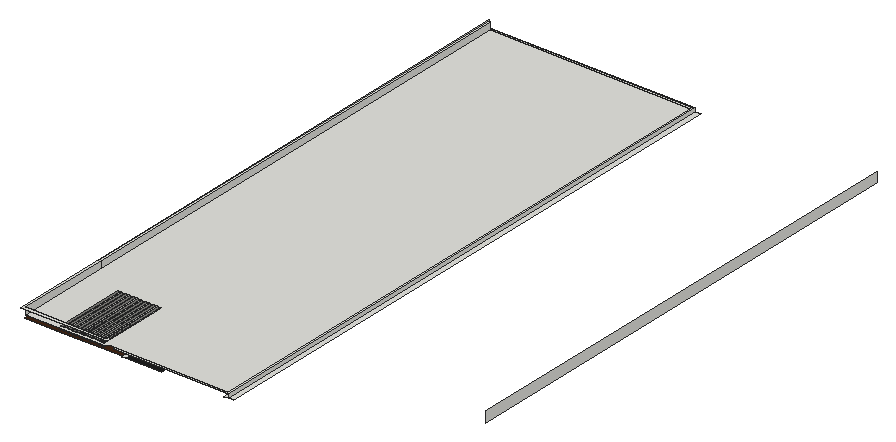
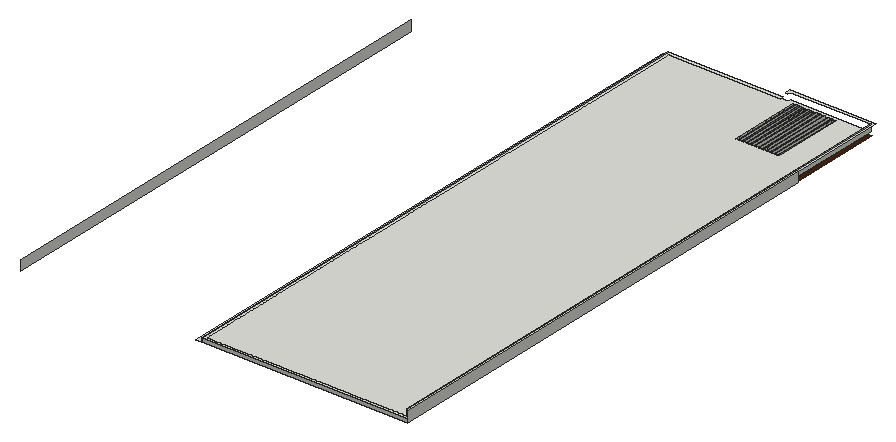
# SketchUp Ruby script. Lengths in inches.
U = 1.inch
M = Sketchup.active_model
def pt(a) = Geom::Point3d.new(a.map { |v| v * U })
def face(e, loops, mat)
  f = e.add_face(loops[0].map { |a| pt(a) })
  loops[1..].each { |l| e.add_face(l.map { |a| pt(a) }).erase! }
  f.material = f.back_material = mat if mat
  f
end
# faces: each face lists its corners as indices into pts; further lists are holes
def faces(e, pts, list, mat = nil) = list.each { |f| face(e, (f[0].is_a?(Array) ? f : [f]).map { |l| l.map { |i| pts[i] } }, mat) }
# xy, xz, yz: faces in a plane at the given z, y or x. An outline is a flat list of corners, or four numbers for a rectangle; further outlines are holes
def ring(l) = l.size == 4 ? [[l[0], l[1]], [l[2], l[1]], [l[2], l[3]], [l[0], l[3]]] : l.each_slice(2).to_a
def flat(e, list, mat, &to3) = list.each { |f| face(e, (f[0].is_a?(Array) ? f : [f]).map { |l| ring(l).map { |u, v| to3.(u, v) } }, mat) }
def xy(e, z, list, mat = nil) = flat(e, list, mat) { |x, y| [x, y, z] }
def xz(e, y, list, mat = nil) = flat(e, list, mat) { |x, z| [x, y, z] }
def yz(e, x, list, mat = nil) = flat(e, list, mat) { |y, z| [x, y, z] }
def lines(e, pts, list) = list.each { |a, b| e.add_line(pt(pts[a]), pt(pts[b])) }
# prism: a flat outline (further loops are holes) pulled along v
def prism(e, loops, v, mat = nil)
  f = face(e, loops, mat); d = Geom::Vector3d.new(v.map { |x| x * U })
  f.pushpull(f.normal.samedirection?(d) ? d.length : -d.length)
end
def box(e, o, s, mat = nil) = prism(e, [[o, [o[0] + s[0], o[1], o[2]], [o[0] + s[0], o[1] + s[1], o[2]], [o[0], o[1] + s[1], o[2]]]], [0, 0, s[2]], mat)
def at(x, y, z, deg = 0) = Geom::Transformation.translation(pt([x, y, z])) * Geom::Transformation.rotation(ORIGIN, Z_AXIS, deg.degrees)
def axes(o, x, y, z) = Geom::Transformation.new([*x, 0, *y, 0, *z, 0, *pt(o).to_a, 1])
def part(name) = M.definitions.add(name)
# library, detail: a bought-in or finely detailed component or shape, given as its bounding box
def library(name, o, s) = part(name).tap { |d| box(d.entities, o, s) }
def detail(e, o, s) = box(e.add_group.entities, o, s)
def put(e, d, t, mat = nil) = e.add_instance(d, t).tap { |i| i.material = mat if mat }
def group(e, t, mat = nil) = e.add_group.tap { |g| g.transformation = t; g.material = mat if mat }.entities
root = M.entities
M.materials.add("[Color M08]").color = [30, 30, 30]
M.materials.add("[Field Square Tile]").color = [211, 167, 108]
M.materials.add("[Granite Light Gray]").color = [149, 148, 144]
M.materials.add("[Wood Veneer 01]").color = [66, 38, 20]
xy(root,380.5,[[2434.04,2346.71,2434.04,3661.44,1986.28,3661.44,1986.28,2597.8,2202.28,2597.8,2202.28,2562.82,1976.47,2562.82,1976.47,3671.25,2443.85,3671.25,2443.85,2346.71],[2202.28,2346.71,2211.2,2425.46],[2443.85,2346.71,2455.66,3671.25],[2202.28,2425.46,2202.28,2597.8,1986.28,2597.8,1986.28,3661.44,2434.04,3661.44,2434.04,2425.46,2387.27,2425.46,2387.27,2532.83,2291.96,2532.83,2291.96,2573.65,2211.2,2573.65,2211.2,2532.83,2202.58,2532.83,2202.58,2425.46],[2202.58,2425.46,2211.2,2532.83],
  [2291.96,2425.46,2387.27,2532.83],[2211.2,2532.83,2291.96,2573.65]])
xy(root,380.5,[[2211.2,2346.71,2291.96,2532.83]],"[Color M08]")
xy(root,380.5,[[[1981.3,2347.9,2053.23,2562.82],[2038.08,2501.63,2039.6,2502.01,2040.98,2502.76,2042.11,2503.84,2042.92,2505.18,2043.35,2506.6875,2043.39,2508.25,2043.01,2509.78,2042.26,2511.15,2041.17,2512.28,2039.83,2513.09,2038.33,2513.53,2036.76,2513.56,2035.24,2513.19,2033.87,2512.43,2032.74,2511.35,2031.93,2510.01,2031.49,2508.5,2031.46,2506.9375,2031.83,2505.41,2032.59,2504.04,2033.67,2502.91,2035.01,2502.1,2036.52,2501.66],[2038.08,2441.63,2039.6,2442.01,2040.98,2442.76,2042.11,2443.84,2042.92,2445.18,2043.35,2446.6875,2043.39,2448.25,2043.01,2449.78,2042.26,2451.15,2041.17,2452.28,2039.83,2453.09,2038.33,2453.53,2036.76,2453.56,2035.24,2453.19,2033.87,2452.43,2032.74,2451.35,2031.93,2450.01,2031.49,2448.5,2031.46,2446.9375,2031.83,2445.41,2032.59,2444.04,2033.67,2442.91,2035.01,2442.1,2036.52,2441.66],[2038.08,2389.88,2039.6,2390.26,2040.98,2391.01,2042.11,2392.09,2042.92,2393.43,2043.35,2394.9375,2043.39,2396.5,2043.01,2398.03,2042.26,2399.4,2041.17,2400.53,2039.83,2401.34,2038.33,2401.78,2036.76,2401.81,2035.24,2401.44,2033.87,2400.68,2032.74,2399.6,2031.93,2398.26,2031.49,2396.75,2031.46,2395.1875,2031.83,2393.66,2032.59,2392.29,2033.67,2391.16,2035.01,2390.35,2036.52,2389.91],[2038.08,2359.13,2039.6,2359.51,2040.98,2360.26,2042.11,2361.34,2042.92,2362.68,2043.35,2364.1875,2043.39,2365.75,2043.01,2367.28,2042.26,2368.65,2041.17,2369.78,2039.83,2370.59,2038.33,2371.03,2036.76,2371.06,2035.24,2370.69,2033.87,2369.93,2032.74,2368.85,2031.93,2367.51,2031.49,2366,2031.46,2364.4375,2031.83,2362.91,2032.59,2361.54,2033.67,2360.41,2035.01,2359.6,2036.52,2359.16],[1998.33,2501.63,1999.85,2502.01,2001.23,2502.76,2002.36,2503.84,2003.17,2505.18,2003.6,2506.6875,2003.64,2508.25,2003.26,2509.78,2002.51,2511.15,2001.42,2512.28,2000.08,2513.09,1998.58,2513.53,1997.01,2513.56,1995.49,2513.19,1994.12,2512.43,1992.99,2511.35,1992.18,2510.01,1991.74,2508.5,1991.71,2506.9375,1992.08,2505.41,1992.84,2504.04,1993.92,2502.91,1995.26,2502.1,1996.77,2501.66],[1998.33,2441.63,1999.85,2442.01,2001.23,2442.76,2002.36,2443.84,2003.17,2445.18,2003.6,2446.6875,2003.64,2448.25,2003.26,2449.78,2002.51,2451.15,2001.42,2452.28,2000.08,2453.09,1998.58,2453.53,1997.01,2453.56,1995.49,2453.19,1994.12,2452.43,1992.99,2451.35,1992.18,2450.01,1991.74,2448.5,1991.71,2446.9375,1992.08,2445.41,1992.84,2444.04,1993.92,2442.91,1995.26,2442.1,1996.77,2441.66],[1998.33,2389.88,1999.85,2390.26,2001.23,2391.01,2002.36,2392.09,2003.17,2393.43,2003.6,2394.9375,2003.64,2396.5,2003.26,2398.03,2002.51,2399.4,2001.42,2400.53,2000.08,2401.34,1998.58,2401.78,1997.01,2401.81,1995.49,2401.44,1994.12,2400.68,1992.99,2399.6,1992.18,2398.26,1991.74,2396.75,1991.71,2395.1875,1992.08,2393.66,1992.84,2392.29,1993.92,2391.16,1995.26,2390.35,1996.77,2389.91],[1998.33,2359.13,1999.85,2359.51,2001.23,2360.26,2002.36,2361.34,2003.17,2362.68,2003.6,2364.1875,2003.64,2365.75,2003.26,2367.28,2002.51,2368.65,2001.42,2369.78,2000.08,2370.59,1998.58,2371.03,1997.01,2371.06,1995.49,2370.69,1994.12,2369.93,1992.99,2368.85,1992.18,2367.51,1991.74,2366,1991.71,2364.4375,1992.08,2362.91,1992.84,2361.54,1993.92,2360.41,1995.26,2359.6,1996.77,2359.16]],[[2053.23,2347.9,2202.28,2562.82],[2148.68,2355.06,2154.93,2516.12],[2139.56,2355.06,2145.81,2516.12],[2130.43,2355.06,2136.68,2516.12],[2121.31,2355.06,2127.56,2516.12],[2112.18,2355.06,2118.43,2516.12],[2103.06,2355.06,2109.31,2516.12],[2093.93,2355.06,2100.18,2516.12],[2084.81,2355.06,2091.06,2516.12],[2075.68,2355.06,2081.93,2516.12],[2066.56,2355.06,2072.81,2516.12],[2057.43,2355.06,2063.68,2516.12]]],"[Wood Veneer 01]")
xy(root,381.875,[[1998.33,2389.88,1996.77,2389.91,1995.26,2390.35,1993.92,2391.16,1992.84,2392.29,1992.08,2393.66,1991.71,2395.1875,1991.74,2396.75,1992.18,2398.26,1992.99,2399.6,1994.12,2400.68,1995.49,2401.44,1997.01,2401.81,1998.58,2401.78,2000.08,2401.34,2001.42,2400.53,2002.51,2399.4,2003.26,2398.03,2003.64,2396.5,2003.6,2394.9375,2003.17,2393.43,2002.36,2392.09,2001.23,2391.01,1999.85,2390.26],[2038.08,2389.88,2036.52,2389.91,2035.01,2390.35,2033.67,2391.16,2032.59,2392.29,2031.83,2393.66,2031.46,2395.1875,2031.49,2396.75,2031.93,2398.26,2032.74,2399.6,2033.87,2400.68,2035.24,2401.44,2036.76,2401.81,2038.33,2401.78,2039.83,2401.34,2041.17,2400.53,2042.26,2399.4,2043.01,2398.03,2043.39,2396.5,2043.35,2394.9375,2042.92,2393.43,2042.11,2392.09,2040.98,2391.01,2039.6,2390.26],[1998.33,2441.63,1996.77,2441.66,1995.26,2442.1,1993.92,2442.91,1992.84,2444.04,1992.08,2445.41,1991.71,2446.9375,1991.74,2448.5,1992.18,2450.01,1992.99,2451.35,1994.12,2452.43,1995.49,2453.19,1997.01,2453.56,1998.58,2453.53,2000.08,2453.09,2001.42,2452.28,2002.51,2451.15,2003.26,2449.78,2003.64,2448.25,2003.6,2446.6875,2003.17,2445.18,2002.36,2443.84,2001.23,2442.76,1999.85,2442.01],[2038.08,2441.63,2036.52,2441.66,2035.01,2442.1,2033.67,2442.91,2032.59,2444.04,2031.83,2445.41,2031.46,2446.9375,2031.49,2448.5,2031.93,2450.01,2032.74,2451.35,2033.87,2452.43,2035.24,2453.19,2036.76,2453.56,2038.33,2453.53,2039.83,2453.09,2041.17,2452.28,2042.26,2451.15,2043.01,2449.78,2043.39,2448.25,2043.35,2446.6875,2042.92,2445.18,2042.11,2443.84,2040.98,2442.76,2039.6,2442.01],[1998.33,2501.63,1996.77,2501.66,1995.26,2502.1,1993.92,2502.91,1992.84,2504.04,1992.08,2505.41,1991.71,2506.9375,1991.74,2508.5,1992.18,2510.01,1992.99,2511.35,1994.12,2512.43,1995.49,2513.19,1997.01,2513.56,1998.58,2513.53,2000.08,2513.09,2001.42,2512.28,2002.51,2511.15,2003.26,2509.78,2003.64,2508.25,2003.6,2506.6875,2003.17,2505.18,2002.36,2503.84,2001.23,2502.76,1999.85,2502.01],
  [2038.08,2501.63,2036.52,2501.66,2035.01,2502.1,2033.67,2502.91,2032.59,2504.04,2031.83,2505.41,2031.46,2506.9375,2031.49,2508.5,2031.93,2510.01,2032.74,2511.35,2033.87,2512.43,2035.24,2513.19,2036.76,2513.56,2038.33,2513.53,2039.83,2513.09,2041.17,2512.28,2042.26,2511.15,2043.01,2509.78,2043.39,2508.25,2043.35,2506.6875,2042.92,2505.18,2042.11,2503.84,2040.98,2502.76,2039.6,2502.01]],"[Field Square Tile]")
xy(root,388.625,[[[1982.81,2346.49,2166.13,2346.49,2166.13,2353.05,2437.5,2353.05,2437.5,3664.91,1982.81,3664.91],[2057.43,2355.06,2063.68,2516.12],[2066.56,2355.06,2072.81,2516.12],[2075.68,2355.06,2081.93,2516.12],[2084.81,2355.06,2091.06,2516.12],[2093.93,2355.06,2100.18,2516.12],[2103.06,2355.06,2109.31,2516.12],[2112.18,2355.06,2118.43,2516.12],[2121.31,2355.06,2127.56,2516.12],[2130.43,2355.06,2136.68,2516.12],[2139.56,2355.06,2145.81,2516.12],[2148.68,2355.06,2154.93,2516.12]],[2183.1875,2346.71,2443.85,2346.71,2443.85,3671.25,1976.47,3671.25,1982.81,3664.91,2437.5,3664.91,2437.5,2353.05,2183.1875,2353.05]])
xy(root,403.8125,[[1976.47,2340.15,2172.48,2340.15,2172.48,2353.05,2166.13,2353.05,2166.13,2346.49,1982.81,2346.49,1982.81,3664.91,1976.47,3671.25]])
xz(root,2516.12,[[2057.43,380.5,2063.68,388.625],[2066.56,380.5,2072.81,388.625],[2075.68,380.5,2081.93,388.625],[2084.81,380.5,2091.06,388.625],[2093.93,380.5,2100.18,388.625],
  [2103.06,380.5,2109.31,388.625],[2112.18,380.5,2118.43,388.625],[2121.31,380.5,2127.56,388.625],[2130.43,380.5,2136.68,388.625],[2139.56,380.5,2145.81,388.625],
  [2148.68,380.5,2154.93,388.625]],"[Granite Light Gray]")
xz(root,3671.25,[[1976.47,380.5,2443.85,388.625]])
yz(root,1976.47,[[2562.82,380.5,3671.25,403.8125]])
yz(root,1982.81,[[2346.49,388.625,2562.82,403.8125],[2562.82,388.625,3664.91,403.8125]])
yz(root,2057.43,[[2355.06,380.5,2516.12,388.625]],"[Granite Light Gray]")
yz(root,2063.68,[[2355.06,380.5,2516.12,388.625]])
yz(root,2066.56,[[2355.06,380.5,2516.12,388.625]],"[Granite Light Gray]")
yz(root,2072.81,[[2355.06,380.5,2516.12,388.625]])
yz(root,2075.68,[[2355.06,380.5,2516.12,388.625]],"[Granite Light Gray]")
yz(root,2081.93,[[2355.06,380.5,2516.12,388.625]])
yz(root,2084.81,[[2355.06,380.5,2516.12,388.625]],"[Granite Light Gray]")
yz(root,2091.06,[[2355.06,380.5,2516.12,388.625]])
yz(root,2093.93,[[2355.06,380.5,2516.12,388.625]],"[Granite Light Gray]")
yz(root,2100.18,[[2355.06,380.5,2516.12,388.625]])
yz(root,2103.06,[[2355.06,380.5,2516.12,388.625]],"[Granite Light Gray]")
yz(root,2109.31,[[2355.06,380.5,2516.12,388.625]])
yz(root,2112.18,[[2355.06,380.5,2516.12,388.625]],"[Granite Light Gray]")
yz(root,2118.43,[[2355.06,380.5,2516.12,388.625]])
yz(root,2121.31,[[2355.06,380.5,2516.12,388.625]],"[Granite Light Gray]")
yz(root,2127.56,[[2355.06,380.5,2516.12,388.625]])
yz(root,2130.43,[[2355.06,380.5,2516.12,388.625]],"[Granite Light Gray]")
yz(root,2136.68,[[2355.06,380.5,2516.12,388.625]])
yz(root,2139.56,[[2355.06,380.5,2516.12,388.625]],"[Granite Light Gray]")
yz(root,2145.81,[[2355.06,380.5,2516.12,388.625]])
yz(root,2148.68,[[2355.06,380.5,2516.12,388.625]],"[Granite Light Gray]")
yz(root,2154.93,[[2355.06,380.5,2516.12,388.625]])
yz(root,2443.85,[[2346.71,380.5,3671.25,388.625]])
yz(root,2855.22,[[2562.82,380.5,3671.25,403.8125]])
p = [[1996.77,2389.91,380.5],[1995.26,2390.35,380.5],[1995.26,2390.35,381.875],[1996.77,2389.91,381.875],[1998.33,2389.88,380.5],[1998.33,2389.88,381.875],
  [1999.85,2390.26,380.5],[1999.85,2390.26,381.875],[2036.52,2389.91,380.5],[2035.01,2390.35,380.5],[2035.01,2390.35,381.875],[2036.52,2389.91,381.875],
  [2038.08,2389.88,380.5],[2038.08,2389.88,381.875],[2039.6,2390.26,380.5],[2039.6,2390.26,381.875],[2001.23,2391.01,380.5],[2001.23,2391.01,381.875],
  [2040.98,2391.01,380.5],[2040.98,2391.01,381.875],[1993.92,2391.16,380.5],[1993.92,2391.16,381.875],[2033.67,2391.16,380.5],[2033.67,2391.16,381.875],
  [2002.36,2392.09,380.5],[2002.36,2392.09,381.875],[2042.11,2392.09,380.5],[2042.11,2392.09,381.875],[1992.84,2392.29,380.5],[1992.84,2392.29,381.875],
  [2032.59,2392.29,380.5],[2032.59,2392.29,381.875],[2003.17,2393.43,380.5],[2003.17,2393.43,381.875],[2042.92,2393.43,380.5],[2042.92,2393.43,381.875],
  [1992.08,2393.66,380.5],[1992.08,2393.66,381.875],[2031.83,2393.66,380.5],[2031.83,2393.66,381.875],[2003.6,2394.9375,380.5],[2003.6,2394.9375,381.875],
  [2043.35,2394.9375,380.5],[2043.35,2394.9375,381.875],[1991.71,2395.1875,380.5],[1991.71,2395.1875,381.875],[2031.46,2395.1875,380.5],[2031.46,2395.1875,381.875],
  [2003.64,2396.5,380.5],[2003.64,2396.5,381.875],[2043.39,2396.5,380.5],[2043.39,2396.5,381.875],[1991.74,2396.75,380.5],[1991.74,2396.75,381.875],
  [2031.49,2396.75,380.5],[2031.49,2396.75,381.875],[2003.26,2398.03,380.5],[2003.26,2398.03,381.875],[2043.01,2398.03,380.5],[2043.01,2398.03,381.875],
  [1992.18,2398.26,380.5],[1992.18,2398.26,381.875],[2031.93,2398.26,380.5],[2031.93,2398.26,381.875],[2002.51,2399.4,380.5],[2002.51,2399.4,381.875],
  [2042.26,2399.4,380.5],[2042.26,2399.4,381.875],[1992.99,2399.6,380.5],[1992.99,2399.6,381.875],[2032.74,2399.6,380.5],[2032.74,2399.6,381.875],
  [2001.42,2400.53,380.5],[2001.42,2400.53,381.875],[2041.17,2400.53,380.5],[2041.17,2400.53,381.875],[1994.12,2400.68,380.5],[1994.12,2400.68,381.875],
  [2033.87,2400.68,380.5],[2033.87,2400.68,381.875],[2000.08,2401.34,380.5],[2000.08,2401.34,381.875],[2039.83,2401.34,380.5],[2039.83,2401.34,381.875],
  [1995.49,2401.44,380.5],[1995.49,2401.44,381.875],[2035.24,2401.44,380.5],[2035.24,2401.44,381.875],[1998.58,2401.78,380.5],[1998.58,2401.78,381.875],
  [2038.33,2401.78,380.5],[2038.33,2401.78,381.875],[1997.01,2401.81,380.5],[1997.01,2401.81,381.875],[2036.76,2401.81,380.5],[2036.76,2401.81,381.875],
  [1998.33,2441.63,380.5],[1996.77,2441.66,380.5],[1996.77,2441.66,381.875],[1998.33,2441.63,381.875],[1999.85,2442.01,380.5],[1999.85,2442.01,381.875],
  [2038.08,2441.63,380.5],[2036.52,2441.66,380.5],[2036.52,2441.66,381.875],[2038.08,2441.63,381.875],[2039.6,2442.01,380.5],[2039.6,2442.01,381.875],
  [1995.26,2442.1,380.5],[1995.26,2442.1,381.875],[2035.01,2442.1,380.5],[2035.01,2442.1,381.875],[2001.23,2442.76,380.5],[2001.23,2442.76,381.875],
  [2040.98,2442.76,380.5],[2040.98,2442.76,381.875],[1993.92,2442.91,380.5],[1993.92,2442.91,381.875],[2033.67,2442.91,380.5],[2033.67,2442.91,381.875],
  [2002.36,2443.84,380.5],[2002.36,2443.84,381.875],[2042.11,2443.84,380.5],[2042.11,2443.84,381.875],[1992.84,2444.04,380.5],[1992.84,2444.04,381.875],
  [2032.59,2444.04,380.5],[2032.59,2444.04,381.875],[2003.17,2445.18,380.5],[2003.17,2445.18,381.875],[2042.92,2445.18,380.5],[2042.92,2445.18,381.875],
  [1992.08,2445.41,380.5],[1992.08,2445.41,381.875],[2031.83,2445.41,380.5],[2031.83,2445.41,381.875],[2003.6,2446.6875,380.5],[2003.6,2446.6875,381.875],
  [2043.35,2446.6875,380.5],[2043.35,2446.6875,381.875],[1991.71,2446.9375,380.5],[1991.71,2446.9375,381.875],[2031.46,2446.9375,380.5],[2031.46,2446.9375,381.875],
  [2003.64,2448.25,380.5],[2003.64,2448.25,381.875],[2043.39,2448.25,380.5],[2043.39,2448.25,381.875],[1991.74,2448.5,380.5],[1991.74,2448.5,381.875],
  [2031.49,2448.5,380.5],[2031.49,2448.5,381.875],[2003.26,2449.78,380.5],[2003.26,2449.78,381.875],[2043.01,2449.78,380.5],[2043.01,2449.78,381.875],
  [1992.18,2450.01,380.5],[1992.18,2450.01,381.875],[2031.93,2450.01,380.5],[2031.93,2450.01,381.875],[2002.51,2451.15,380.5],[2002.51,2451.15,381.875],
  [2042.26,2451.15,380.5],[2042.26,2451.15,381.875],[1992.99,2451.35,380.5],[1992.99,2451.35,381.875],[2032.74,2451.35,380.5],[2032.74,2451.35,381.875],
  [2001.42,2452.28,380.5],[2001.42,2452.28,381.875],[2041.17,2452.28,380.5],[2041.17,2452.28,381.875],[1994.12,2452.43,380.5],[1994.12,2452.43,381.875],
  [2033.87,2452.43,380.5],[2033.87,2452.43,381.875],[2000.08,2453.09,380.5],[2000.08,2453.09,381.875],[2039.83,2453.09,380.5],[2039.83,2453.09,381.875],
  [1995.49,2453.19,380.5],[1995.49,2453.19,381.875],[2035.24,2453.19,380.5],[2035.24,2453.19,381.875],[1998.58,2453.53,380.5],[1998.58,2453.53,381.875],
  [2038.33,2453.53,380.5],[2038.33,2453.53,381.875],[1997.01,2453.56,380.5],[1997.01,2453.56,381.875],[2036.76,2453.56,380.5],[2036.76,2453.56,381.875],
  [1998.33,2501.63,380.5],[1996.77,2501.66,380.5],[1996.77,2501.66,381.875],[1998.33,2501.63,381.875],[1999.85,2502.01,380.5],[1999.85,2502.01,381.875],
  [2038.08,2501.63,380.5],[2036.52,2501.66,380.5],[2036.52,2501.66,381.875],[2038.08,2501.63,381.875],[2039.6,2502.01,380.5],[2039.6,2502.01,381.875],
  [1995.26,2502.1,380.5],[1995.26,2502.1,381.875],[2035.01,2502.1,380.5],[2035.01,2502.1,381.875],[2001.23,2502.76,380.5],[2001.23,2502.76,381.875],
  [2040.98,2502.76,380.5],[2040.98,2502.76,381.875],[1993.92,2502.91,380.5],[1993.92,2502.91,381.875],[2033.67,2502.91,380.5],[2033.67,2502.91,381.875],
  [2002.36,2503.84,380.5],[2002.36,2503.84,381.875],[2042.11,2503.84,380.5],[2042.11,2503.84,381.875],[1992.84,2504.04,380.5],[1992.84,2504.04,381.875],
  [2032.59,2504.04,380.5],[2032.59,2504.04,381.875],[2003.17,2505.18,380.5],[2003.17,2505.18,381.875],[2042.92,2505.18,380.5],[2042.92,2505.18,381.875],
  [1992.08,2505.41,380.5],[1992.08,2505.41,381.875],[2031.83,2505.41,380.5],[2031.83,2505.41,381.875],[2003.6,2506.6875,380.5],[2003.6,2506.6875,381.875],
  [2043.35,2506.6875,380.5],[2043.35,2506.6875,381.875],[1991.71,2506.9375,380.5],[1991.71,2506.9375,381.875],[2031.46,2506.9375,380.5],[2031.46,2506.9375,381.875],
  [2003.64,2508.25,380.5],[2003.64,2508.25,381.875],[2043.39,2508.25,380.5],[2043.39,2508.25,381.875],[1991.74,2508.5,380.5],[1991.74,2508.5,381.875],
  [2031.49,2508.5,380.5],[2031.49,2508.5,381.875],[2003.26,2509.78,380.5],[2003.26,2509.78,381.875],[2043.01,2509.78,380.5],[2043.01,2509.78,381.875],
  [1992.18,2510.01,380.5],[1992.18,2510.01,381.875],[2031.93,2510.01,380.5],[2031.93,2510.01,381.875],[2002.51,2511.15,380.5],[2002.51,2511.15,381.875],
  [2042.26,2511.15,380.5],[2042.26,2511.15,381.875],[1992.99,2511.35,380.5],[1992.99,2511.35,381.875],[2032.74,2511.35,380.5],[2032.74,2511.35,381.875],
  [2001.42,2512.28,380.5],[2001.42,2512.28,381.875],[2041.17,2512.28,380.5],[2041.17,2512.28,381.875],[1994.12,2512.43,380.5],[1994.12,2512.43,381.875],
  [2033.87,2512.43,380.5],[2033.87,2512.43,381.875],[2000.08,2513.09,380.5],[2000.08,2513.09,381.875],[2039.83,2513.09,380.5],[2039.83,2513.09,381.875],
  [1995.49,2513.19,380.5],[1995.49,2513.19,381.875],[2035.24,2513.19,380.5],[2035.24,2513.19,381.875],[1998.58,2513.53,380.5],[1998.58,2513.53,381.875],
  [2038.33,2513.53,380.5],[2038.33,2513.53,381.875],[1997.01,2513.56,380.5],[1997.01,2513.56,381.875],[2036.76,2513.56,380.5],[2036.76,2513.56,381.875],
  [1982.81,3664.91,388.625],[1976.47,3671.25,388.625],[1976.47,3671.25,403.8125],[1982.81,3664.91,403.8125]]
faces(root,p,[[0,1,2,3],[4,0,3,5],[6,4,5,7],[8,9,10,11],[12,8,11,13],[14,12,13,15],[16,6,7,17],[18,14,15,19],
  [1,20,21,2],[9,22,23,10],[24,16,17,25],[26,18,19,27],[20,28,29,21],[22,30,31,23],[32,24,25,33],[34,26,27,35],
  [28,36,37,29],[30,38,39,31],[40,32,33,41],[42,34,35,43],[36,44,45,37],[38,46,47,39],[48,40,41,49],[50,42,43,51],
  [44,52,53,45],[46,54,55,47],[56,48,49,57],[58,50,51,59],[52,60,61,53],[54,62,63,55],[64,56,57,65],[66,58,59,67],
  [60,68,69,61],[62,70,71,63],[72,64,65,73],[74,66,67,75],[68,76,77,69],[70,78,79,71],[80,72,73,81],[82,74,75,83],
  [76,84,85,77],[78,86,87,79],[88,80,81,89],[90,82,83,91],[84,92,93,85],[86,94,95,87],[92,88,89,93],[94,90,91,95],
  [96,97,98,99],[100,96,99,101],[102,103,104,105],[106,102,105,107],[97,108,109,98],[103,110,111,104],[112,100,101,113],[114,106,107,115],
  [108,116,117,109],[110,118,119,111],[120,112,113,121],[122,114,115,123],[116,124,125,117],[118,126,127,119],[128,120,121,129],[130,122,123,131],
  [124,132,133,125],[126,134,135,127],[136,128,129,137],[138,130,131,139],[132,140,141,133],[134,142,143,135],[144,136,137,145],[146,138,139,147],
  [140,148,149,141],[142,150,151,143],[152,144,145,153],[154,146,147,155],[148,156,157,149],[150,158,159,151],[160,152,153,161],[162,154,155,163],
  [156,164,165,157],[158,166,167,159],[168,160,161,169],[170,162,163,171],[164,172,173,165],[166,174,175,167],[176,168,169,177],[178,170,171,179],
  [172,180,181,173],[174,182,183,175],[184,176,177,185],[186,178,179,187],[180,188,189,181],[182,190,191,183],[188,184,185,189],[190,186,187,191],
  [192,193,194,195],[196,192,195,197],[198,199,200,201],[202,198,201,203],[193,204,205,194],[199,206,207,200],[208,196,197,209],[210,202,203,211],
  [204,212,213,205],[206,214,215,207],[216,208,209,217],[218,210,211,219],[212,220,221,213],[214,222,223,215],[224,216,217,225],[226,218,219,227],
  [220,228,229,221],[222,230,231,223],[232,224,225,233],[234,226,227,235],[228,236,237,229],[230,238,239,231],[240,232,233,241],[242,234,235,243],
  [236,244,245,237],[238,246,247,239],[248,240,241,249],[250,242,243,251],[244,252,253,245],[246,254,255,247],[256,248,249,257],[258,250,251,259],
  [252,260,261,253],[254,262,263,255],[264,256,257,265],[266,258,259,267],[260,268,269,261],[262,270,271,263],[272,264,265,273],[274,266,267,275],
  [268,276,277,269],[270,278,279,271],[280,272,273,281],[282,274,275,283],[276,284,285,277],[278,286,287,279],[284,280,281,285],[286,282,283,287]],"[Field Square Tile]")
faces(root,p,[[288,289,290,291]])
